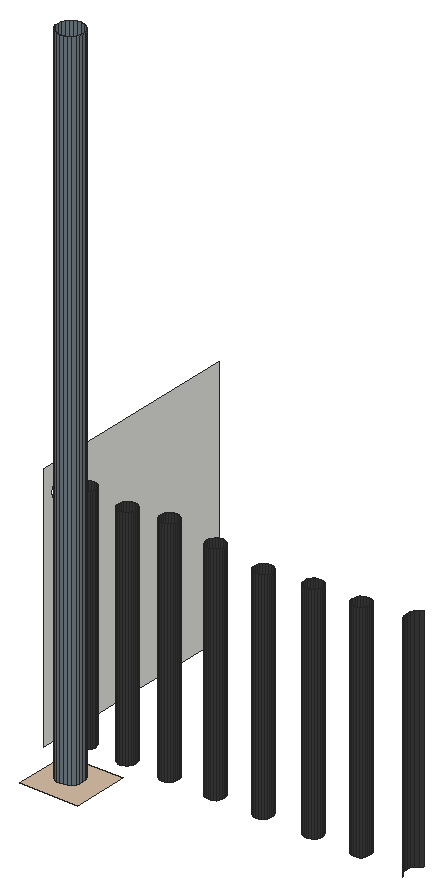
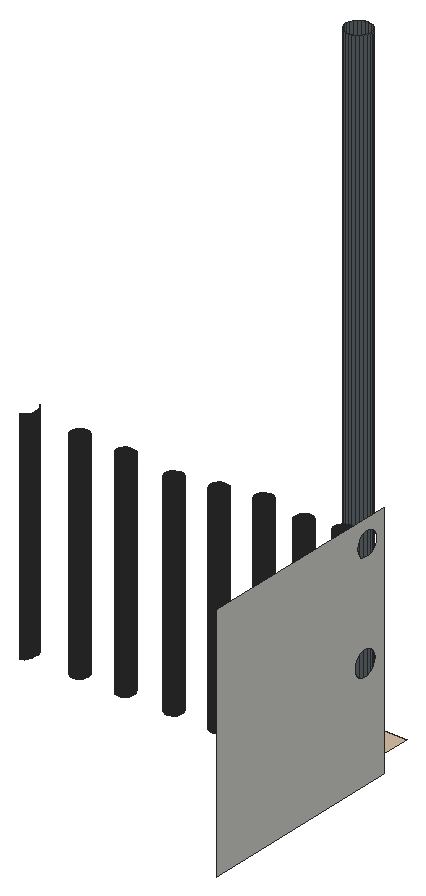
# SketchUp Ruby script. Lengths in inches.
U = 1.inch
M = Sketchup.active_model
def pt(a) = Geom::Point3d.new(a.map { |v| v * U })
def face(e, loops, mat)
  f = e.add_face(loops[0].map { |a| pt(a) })
  loops[1..].each { |l| e.add_face(l.map { |a| pt(a) }).erase! }
  f.material = f.back_material = mat if mat
  f
end
# faces: each face lists its corners as indices into pts; further lists are holes
def faces(e, pts, list, mat = nil) = list.each { |f| face(e, (f[0].is_a?(Array) ? f : [f]).map { |l| l.map { |i| pts[i] } }, mat) }
# xy, xz, yz: faces in a plane at the given z, y or x. An outline is a flat list of corners, or four numbers for a rectangle; further outlines are holes
def ring(l) = l.size == 4 ? [[l[0], l[1]], [l[2], l[1]], [l[2], l[3]], [l[0], l[3]]] : l.each_slice(2).to_a
def flat(e, list, mat, &to3) = list.each { |f| face(e, (f[0].is_a?(Array) ? f : [f]).map { |l| ring(l).map { |u, v| to3.(u, v) } }, mat) }
def xy(e, z, list, mat = nil) = flat(e, list, mat) { |x, y| [x, y, z] }
def xz(e, y, list, mat = nil) = flat(e, list, mat) { |x, z| [x, y, z] }
def yz(e, x, list, mat = nil) = flat(e, list, mat) { |y, z| [x, y, z] }
def lines(e, pts, list) = list.each { |a, b| e.add_line(pt(pts[a]), pt(pts[b])) }
# prism: a flat outline (further loops are holes) pulled along v
def prism(e, loops, v, mat = nil)
  f = face(e, loops, mat); d = Geom::Vector3d.new(v.map { |x| x * U })
  f.pushpull(f.normal.samedirection?(d) ? d.length : -d.length)
end
def box(e, o, s, mat = nil) = prism(e, [[o, [o[0] + s[0], o[1], o[2]], [o[0] + s[0], o[1] + s[1], o[2]], [o[0], o[1] + s[1], o[2]]]], [0, 0, s[2]], mat)
def at(x, y, z, deg = 0) = Geom::Transformation.translation(pt([x, y, z])) * Geom::Transformation.rotation(ORIGIN, Z_AXIS, deg.degrees)
def axes(o, x, y, z) = Geom::Transformation.new([*x, 0, *y, 0, *z, 0, *pt(o).to_a, 1])
def part(name) = M.definitions.add(name)
# library, detail: a bought-in or finely detailed component or shape, given as its bounding box
def library(name, o, s) = part(name).tap { |d| box(d.entities, o, s) }
def detail(e, o, s) = box(e.add_group.entities, o, s)
def put(e, d, t, mat = nil) = e.add_instance(d, t).tap { |i| i.material = mat if mat }
def group(e, t, mat = nil) = e.add_group.tap { |g| g.transformation = t; g.material = mat if mat }.entities
root = M.entities
M.materials.add("[Color M07]").color = [58, 58, 58]
M.materials.add("[Formica Laminate Light]").color = [213, 189, 164]
M.materials.add("[Formica Speckled Grey]").color = [112, 125, 132]
xy(root,479.18,[[50.05,85.59,49.68,85.64,49.33,85.79,49.03,86.02,48.81,86.3125,48.66,86.66,48.61,87.03,48.66,87.4,48.81,87.75,49.03,88.05,49.33,88.28,49.68,88.42,50.05,88.47,50.42,88.42,50.77,88.28,51.07,88.05,51.3,87.75,51.4375,87.4,51.49,87.03,51.4375,86.66,51.3,86.3125,51.07,86.02,50.77,85.79,50.42,85.64],[47.49,91.47,47.23,91.5,46.99,91.6,46.78,91.76,46.62,91.97,46.52,92.21,46.49,92.47,46.52,92.73,46.62,92.97,46.78,93.18,46.99,93.33,47.23,93.43,47.49,93.47,47.74,93.43,47.99,93.33,48.19,93.18,48.35,92.97,48.45,92.73,48.49,92.47,48.45,92.21,48.35,91.97,48.19,91.76,47.99,91.6,47.74,91.5],[52.05,91.47,51.79,91.5,51.55,91.6,51.34,91.76,51.18,91.97,51.08,92.21,51.05,92.47,51.08,92.73,51.18,92.97,51.34,93.18,51.55,93.33,51.79,93.43,52.05,93.47,52.31,93.43,52.55,93.33,52.76,93.18,52.91,92.97,53.01,92.73,53.05,92.47,53.01,92.21,52.91,91.97,52.76,91.76,52.55,91.6,52.31,91.5],[56.74,91.47,56.48,91.5,56.24,91.6,56.03,91.76,55.87,91.97,55.77,92.21,55.74,92.47,55.77,92.73,55.87,92.97,56.03,93.18,56.24,93.33,56.48,93.43,56.74,93.47,56.99,93.43,57.24,93.33,57.44,93.18,57.6,92.97,57.7,92.73,57.74,92.47,57.7,92.21,57.6,91.97,57.44,91.76,57.24,91.6,56.99,91.5],[61.92,91.47,61.66,91.5,61.42,91.6,61.22,91.76,61.06,91.97,60.96,92.21,60.92,92.47,60.96,92.73,61.06,92.97,61.22,93.18,61.42,93.33,61.66,93.43,61.92,93.47,62.18,93.43,62.42,93.33,62.63,93.18,62.79,92.97,62.89,92.73,62.92,92.47,62.89,92.21,62.79,91.97,62.63,91.76,62.42,91.6,62.18,91.5],
  [67.24,91.47,66.98,91.5,66.74,91.6,66.53,91.76,66.37,91.97,66.27,92.21,66.24,92.47,66.27,92.73,66.37,92.97,66.53,93.18,66.74,93.33,66.98,93.43,67.24,93.47,67.49,93.43,67.74,93.33,67.94,93.18,68.1,92.97,68.2,92.73,68.24,92.47,68.2,92.21,68.1,91.97,67.94,91.76,67.74,91.6,67.49,91.5],[72.86,91.47,72.6,91.5,72.36,91.6,72.15,91.76,71.99,91.97,71.89,92.21,71.86,92.47,71.89,92.73,71.99,92.97,72.15,93.18,72.36,93.33,72.6,93.43,72.86,93.47,73.12,93.43,73.36,93.33,73.57,93.18,73.73,92.97,73.83,92.73,73.86,92.47,73.83,92.21,73.73,91.97,73.57,91.76,73.36,91.6,73.12,91.5],[78.17,91.47,77.91,91.5,77.67,91.6,77.47,91.76,77.31,91.97,77.21,92.21,77.17,92.47,77.21,92.73,77.31,92.97,77.47,93.18,77.67,93.33,77.91,93.43,78.17,93.47,78.43,93.43,78.67,93.33,78.88,93.18,79.04,92.97,79.14,92.73,79.17,92.47,79.14,92.21,79.04,91.97,78.88,91.76,78.67,91.6,78.43,91.5]])
xy(root,479.18,[[[47.29,83.48,53.75,89.73],[50.05,85.59,49.68,85.64,49.33,85.79,49.03,86.02,48.81,86.3125,48.66,86.66,48.61,87.03,48.66,87.4,48.81,87.75,49.03,88.05,49.33,88.28,49.68,88.42,50.05,88.47,50.42,88.42,50.77,88.28,51.07,88.05,51.3,87.75,51.4375,87.4,51.49,87.03,51.4375,86.66,51.3,86.3125,51.07,86.02,50.77,85.79,50.42,85.64]]],"[Formica Laminate Light]")
yz(root,44.94,[[[89.73,479.18,114.1,506.99],[92.45,490.42,92.06,490.47,91.7,490.62,91.39,490.86,91.15,491.17,91,491.53,90.95,491.92,91,492.31,91.15,492.67,91.39,492.98,91.7,493.22,92.06,493.37,92.45,493.42,92.84,493.37,93.2,493.22,93.51,492.98,93.75,492.67,93.9,492.31,93.95,491.92,93.9,491.53,93.75,491.17,93.51,490.86,93.2,490.62,92.84,490.47],[92.15,502.86,91.77,502.91,91.43,503.05,91.13,503.28,90.9,503.58,90.76,503.92,90.71,504.3,90.76,504.67,90.9,505.01,91.13,505.3125,91.43,505.54,91.77,505.68,92.15,505.73,92.52,505.68,92.87,505.54,93.16,505.3125,93.39,505.01,93.53,504.67,93.58,504.3,93.53,503.92,93.39,503.58,93.16,503.28,92.87,503.05,92.52,502.91]]])
p = [[49.33,85.79,479.18],[49.68,85.64,479.18],[49.68,85.64,554.07],[49.33,85.79,554.07],[50.05,85.59,479.18],[50.05,85.59,554.07],
  [50.42,85.64,479.18],[50.42,85.64,554.07],[50.77,85.79,479.18],[50.77,85.79,554.07],[50.46,85.66,554.07],[49.03,86.02,479.18],
  [49.03,86.02,554.07],[51.07,86.02,479.18],[51.07,86.02,554.07],[48.81,86.3125,479.18],[48.81,86.3125,554.07],[51.3,86.3125,479.18],
  [51.3,86.3125,554.07],[48.66,86.66,479.18],[48.66,86.66,554.07],[51.4375,86.66,479.18],[51.4375,86.66,554.07],[48.61,87.03,479.18],
  [48.61,87.03,554.07],[51.49,87.03,479.18],[51.49,87.03,554.07],[48.66,87.4,479.18],[48.66,87.4,554.07],[51.4375,87.4,479.18],
  [51.4375,87.4,554.07],[48.81,87.75,479.18],[48.81,87.75,554.07],[51.3,87.75,479.18],[51.3,87.75,554.07],[49.03,88.05,479.18],
  [49.03,88.05,554.07],[51.07,88.05,479.18],[51.07,88.05,554.07],[49.33,88.28,479.18],[49.33,88.28,554.07],[50.77,88.28,479.18],
  [50.77,88.28,554.07],[49.68,88.42,479.18],[49.68,88.42,554.07],[50.42,88.42,479.18],[50.42,88.42,554.07],[50.46,88.4,554.07],
  [50.05,88.47,479.18],[50.05,88.47,554.07],[83.49,91.66,479.18],[83.74,91.33,479.18],[83.74,91.33,504.8],[83.49,91.66,504.8],
  [46.99,91.6,479.18],[47.23,91.5,479.18],[47.23,91.5,505.01],[46.99,91.6,505.01],[47.49,91.47,479.18],[47.49,91.47,505.01],
  [47.74,91.5,479.18],[47.74,91.5,505.01],[47.99,91.6,479.18],[47.99,91.6,505.01],[51.55,91.6,479.18],[51.79,91.5,479.18],
  [51.79,91.5,504.49],[51.55,91.6,504.49],[52.05,91.47,479.18],[52.05,91.47,504.49],[52.31,91.5,479.18],[52.31,91.5,504.49],
  [52.55,91.6,479.18],[52.55,91.6,504.49],[56.24,91.6,479.18],[56.48,91.5,479.18],[56.48,91.5,505.01],[56.24,91.6,505.01],
  [56.74,91.47,479.18],[56.74,91.47,505.01],[56.99,91.5,479.18],[56.99,91.5,505.01],[57.24,91.6,479.18],[57.24,91.6,505.01],
  [61.42,91.6,479.18],[61.66,91.5,479.18],[61.66,91.5,504.3],[61.42,91.6,504.3],[61.92,91.47,479.18],[61.92,91.47,504.3],
  [62.18,91.5,479.18],[62.18,91.5,504.3],[62.42,91.6,479.18],[62.42,91.6,504.3],[66.74,91.6,479.18],[66.98,91.5,479.18],
  [66.98,91.5,503.62],[66.74,91.6,503.62],[67.24,91.47,479.18],[67.24,91.47,503.62],[67.49,91.5,479.18],[67.49,91.5,503.62],
  [67.74,91.6,479.18],[67.74,91.6,503.62],[72.36,91.6,479.18],[72.6,91.5,479.18],[72.6,91.5,504.12],[72.36,91.6,504.12],
  [72.86,91.47,479.18],[72.86,91.47,504.12],[73.12,91.5,479.18],[73.12,91.5,504.12],[73.36,91.6,479.18],[73.36,91.6,504.12],
  [77.67,91.6,479.18],[77.91,91.5,479.18],[77.91,91.5,504.18],[77.67,91.6,504.18],[78.17,91.47,479.18],[78.17,91.47,504.18],
  [78.43,91.5,479.18],[78.43,91.5,504.18],[78.67,91.6,479.18],[78.67,91.6,504.18],[46.78,91.76,479.18],[46.78,91.76,505.01],
  [48.19,91.76,479.18],[48.19,91.76,505.01],[51.34,91.76,479.18],[51.34,91.76,504.49],[52.76,91.76,479.18],[52.76,91.76,504.49],
  [56.03,91.76,479.18],[56.03,91.76,505.01],[57.44,91.76,479.18],[57.44,91.76,505.01],[61.22,91.76,479.18],[61.22,91.76,504.3],
  [62.63,91.76,479.18],[62.63,91.76,504.3],[66.53,91.76,479.18],[66.53,91.76,503.62],[67.94,91.76,479.18],[67.94,91.76,503.62],
  [72.15,91.76,479.18],[72.15,91.76,504.12],[73.57,91.76,479.18],[73.57,91.76,504.12],[77.47,91.76,479.18],[77.47,91.76,504.18],
  [78.88,91.76,479.18],[78.88,91.76,504.18],[83.34,92.03,479.18],[83.34,92.03,504.8],[46.62,91.97,479.18],[46.62,91.97,505.01],
  [48.35,91.97,479.18],[48.35,91.97,505.01],[51.18,91.97,479.18],[51.18,91.97,504.49],[52.91,91.97,479.18],[52.91,91.97,504.49],
  [55.87,91.97,479.18],[55.87,91.97,505.01],[57.6,91.97,479.18],[57.6,91.97,505.01],[61.06,91.97,479.18],[61.06,91.97,504.3],
  [62.79,91.97,479.18],[62.79,91.97,504.3],[66.37,91.97,479.18],[66.37,91.97,503.62],[68.1,91.97,479.18],[68.1,91.97,503.62],
  [71.99,91.97,479.18],[71.99,91.97,504.12],[73.73,91.97,479.18],[73.73,91.97,504.12],[77.31,91.97,479.18],[77.31,91.97,504.18],
  [79.04,91.97,479.18],[79.04,91.97,504.18],[46.52,92.21,479.18],[46.52,92.21,505.01],[48.45,92.21,479.18],[48.45,92.21,505.01],
  [51.08,92.21,479.18],[51.08,92.21,504.49],[53.01,92.21,479.18],[53.01,92.21,504.49],[55.77,92.21,479.18],[55.77,92.21,505.01],
  [57.7,92.21,479.18],[57.7,92.21,505.01],[60.96,92.21,479.18],[60.96,92.21,504.3],[62.89,92.21,479.18],[62.89,92.21,504.3],
  [66.27,92.21,479.18],[66.27,92.21,503.62],[68.2,92.21,479.18],[68.2,92.21,503.62],[71.89,92.21,479.18],[71.89,92.21,504.12],
  [73.83,92.21,479.18],[73.83,92.21,504.12],[77.21,92.21,479.18],[77.21,92.21,504.18],[79.14,92.21,479.18],[79.14,92.21,504.18],
  [83.28,92.4375,479.18],[83.28,92.4375,504.8],[46.49,92.47,479.18],[46.49,92.47,505.01],[48.49,92.47,479.18],[48.49,92.47,505.01],
  [51.05,92.47,479.18],[51.05,92.47,504.49],[53.05,92.47,479.18],[53.05,92.47,504.49],[55.74,92.47,479.18],[55.74,92.47,505.01],
  [57.74,92.47,479.18],[57.74,92.47,505.01],[60.92,92.47,479.18],[60.92,92.47,504.3],[62.92,92.47,479.18],[62.92,92.47,504.3],
  [66.24,92.47,479.18],[66.24,92.47,503.62],[68.24,92.47,479.18],[68.24,92.47,503.62],[71.86,92.47,479.18],[71.86,92.47,504.12],
  [73.86,92.47,479.18],[73.86,92.47,504.12],[77.17,92.47,479.18],[77.17,92.47,504.18],[79.17,92.47,479.18],[79.17,92.47,504.18],
  [83.34,92.84,479.18],[83.34,92.84,504.8],[46.52,92.73,479.18],[46.52,92.73,505.01],[48.45,92.73,479.18],[48.45,92.73,505.01],
  [51.08,92.73,479.18],[51.08,92.73,504.49],[53.01,92.73,479.18],[53.01,92.73,504.49],[55.77,92.73,479.18],[55.77,92.73,505.01],
  [57.7,92.73,479.18],[57.7,92.73,505.01],[60.96,92.73,479.18],[60.96,92.73,504.3],[62.89,92.73,479.18],[62.89,92.73,504.3],
  [66.27,92.73,479.18],[66.27,92.73,503.62],[68.2,92.73,479.18],[68.2,92.73,503.62],[71.89,92.73,479.18],[71.89,92.73,504.12],
  [73.83,92.73,479.18],[73.83,92.73,504.12],[77.21,92.73,479.18],[77.21,92.73,504.18],[79.14,92.73,479.18],[79.14,92.73,504.18],
  [46.62,92.97,479.18],[46.62,92.97,505.01],[48.35,92.97,479.18],[48.35,92.97,505.01],[51.18,92.97,479.18],[51.18,92.97,504.49],
  [52.91,92.97,479.18],[52.91,92.97,504.49],[55.87,92.97,479.18],[55.87,92.97,505.01],[57.6,92.97,479.18],[57.6,92.97,505.01],
  [61.06,92.97,479.18],[61.06,92.97,504.3],[62.79,92.97,479.18],[62.79,92.97,504.3],[66.37,92.97,479.18],[66.37,92.97,503.62],
  [68.1,92.97,479.18],[68.1,92.97,503.62],[71.99,92.97,479.18],[71.99,92.97,504.12],[73.73,92.97,479.18],[73.73,92.97,504.12],
  [77.31,92.97,479.18],[77.31,92.97,504.18],[79.04,92.97,479.18],[79.04,92.97,504.18],[83.49,93.22,479.18],[83.49,93.22,504.8],
  [46.78,93.18,479.18],[46.78,93.18,505.01],[48.19,93.18,479.18],[48.19,93.18,505.01],[51.34,93.18,479.18],[51.34,93.18,504.49],
  [52.76,93.18,479.18],[52.76,93.18,504.49],[56.03,93.18,479.18],[56.03,93.18,505.01],[57.44,93.18,479.18],[57.44,93.18,505.01],
  [61.22,93.18,479.18],[61.22,93.18,504.3],[62.63,93.18,479.18],[62.63,93.18,504.3],[66.53,93.18,479.18],[66.53,93.18,503.62],
  [67.94,93.18,479.18],[67.94,93.18,503.62],[72.15,93.18,479.18],[72.15,93.18,504.12],[73.57,93.18,479.18],[73.57,93.18,504.12],
  [77.47,93.18,479.18],[77.47,93.18,504.18],[78.88,93.18,479.18],[78.88,93.18,504.18],[46.99,93.33,479.18],[46.99,93.33,505.01],
  [47.99,93.33,479.18],[47.99,93.33,505.01],[51.55,93.33,479.18],[51.55,93.33,504.49],[52.55,93.33,479.18],[52.55,93.33,504.49],
  [56.24,93.33,479.18],[56.24,93.33,505.01],[57.24,93.33,479.18],[57.24,93.33,505.01],[61.42,93.33,479.18],[61.42,93.33,504.3],
  [62.42,93.33,479.18],[62.42,93.33,504.3],[66.74,93.33,479.18],[66.74,93.33,503.62],[67.74,93.33,479.18],[67.74,93.33,503.62],
  [72.36,93.33,479.18],[72.36,93.33,504.12],[73.36,93.33,479.18],[73.36,93.33,504.12],[77.67,93.33,479.18],[77.67,93.33,504.18],
  [78.67,93.33,479.18],[78.67,93.33,504.18],[83.74,93.54,479.18],[83.74,93.54,504.8],[47.23,93.43,479.18],[47.12,93.39,505.01],
  [47.23,93.43,505.01],[47.74,93.43,479.18],[47.74,93.43,505.01],[47.85,93.39,505.01],[51.79,93.43,479.18],[51.79,93.43,504.49],
  [52.31,93.43,479.18],[52.31,93.43,504.49],[56.48,93.43,479.18],[56.37,93.39,505.01],[56.48,93.43,505.01],[56.99,93.43,479.18],
  [56.99,93.43,505.01],[57.1,93.39,505.01],[61.66,93.43,479.18],[61.66,93.43,504.3],[62.18,93.43,479.18],[62.18,93.43,504.3],
  [66.98,93.43,479.18],[66.98,93.43,503.62],[67.49,93.43,479.18],[67.49,93.43,503.62],[72.6,93.43,479.18],[72.6,93.43,504.12],
  [73.12,93.43,479.18],[73.12,93.43,504.12],[77.91,93.43,479.18],[77.91,93.43,504.18],[78.43,93.43,479.18],[78.43,93.43,504.18],
  [47.49,93.47,479.18],[47.49,93.47,505.01],[52.05,93.47,479.18],[52.05,93.47,504.49],[56.74,93.47,479.18],[56.74,93.47,505.01],
  [61.92,93.47,479.18],[61.92,93.47,504.3],[67.24,93.47,479.18],[67.24,93.47,503.62],[72.86,93.47,479.18],[72.86,93.47,504.12],
  [78.17,93.47,479.18],[78.17,93.47,504.18],[84.0625,93.79,479.18],[84.0625,93.79,504.8]]
faces(root,p,[[0,1,2,3],[1,4,5,2],[4,6,7,5],[6,8,9,10,7],[11,0,3,12],[8,13,14,9],[15,11,12,16],[13,17,18,14],
  [19,15,16,20],[17,21,22,18],[23,19,20,24],[21,25,26,22],[27,23,24,28],[25,29,30,26],[31,27,28,32],[29,33,34,30],
  [35,31,32,36],[33,37,38,34],[39,35,36,40],[37,41,42,38],[43,39,40,44],[41,45,46,47,42],[48,43,44,49],[45,48,49,46]],"[Formica Speckled Grey]")
faces(root,p,[[50,51,52,53],[54,55,56,57],[55,58,59,56],[58,60,61,59],[60,62,63,61],[64,65,66,67],[65,68,69,66],[68,70,71,69],
  [70,72,73,71],[74,75,76,77],[75,78,79,76],[78,80,81,79],[80,82,83,81],[84,85,86,87],[85,88,89,86],[88,90,91,89],
  [90,92,93,91],[94,95,96,97],[95,98,99,96],[98,100,101,99],[100,102,103,101],[104,105,106,107],[105,108,109,106],[108,110,111,109],
  [110,112,113,111],[114,115,116,117],[115,118,119,116],[118,120,121,119],[120,122,123,121],[124,54,57,125],[62,126,127,63],[128,64,67,129],
  [72,130,131,73],[132,74,77,133],[82,134,135,83],[136,84,87,137],[92,138,139,93],[140,94,97,141],[102,142,143,103],[144,104,107,145],
  [112,146,147,113],[148,114,117,149],[122,150,151,123],[152,50,53,153],[154,124,125,155],[126,156,157,127],[158,128,129,159],[130,160,161,131],
  [162,132,133,163],[134,164,165,135],[166,136,137,167],[138,168,169,139],[170,140,141,171],[142,172,173,143],[174,144,145,175],[146,176,177,147],
  [178,148,149,179],[150,180,181,151],[182,154,155,183],[156,184,185,157],[186,158,159,187],[160,188,189,161],[190,162,163,191],[164,192,193,165],
  [194,166,167,195],[168,196,197,169],[198,170,171,199],[172,200,201,173],[202,174,175,203],[176,204,205,177],[206,178,179,207],[180,208,209,181],
  [210,152,153,211],[212,182,183,213],[184,214,215,185],[216,186,187,217],[188,218,219,189],[220,190,191,221],[192,222,223,193],[224,194,195,225],
  [196,226,227,197],[228,198,199,229],[200,230,231,201],[232,202,203,233],[204,234,235,205],[236,206,207,237],[208,238,239,209],[240,210,211,241],
  [242,212,213,243],[214,244,245,215],[246,216,217,247],[218,248,249,219],[250,220,221,251],[222,252,253,223],[254,224,225,255],[226,256,257,227],
  [258,228,229,259],[230,260,261,231],[262,232,233,263],[234,264,265,235],[266,236,237,267],[238,268,269,239],[270,242,243,271],[244,272,273,245],
  [274,246,247,275],[248,276,277,249],[278,250,251,279],[252,280,281,253],[282,254,255,283],[256,284,285,257],[286,258,259,287],[260,288,289,261],
  [290,262,263,291],[264,292,293,265],[294,266,267,295],[268,296,297,269],[298,240,241,299],[300,270,271,301],[272,302,303,273],[304,274,275,305],
  [276,306,307,277],[308,278,279,309],[280,310,311,281],[312,282,283,313],[284,314,315,285],[316,286,287,317],[288,318,319,289],[320,290,291,321],
  [292,322,323,293],[324,294,295,325],[296,326,327,297],[328,300,301,329],[302,330,331,303],[332,304,305,333],[306,334,335,307],[336,308,309,337],
  [310,338,339,311],[340,312,313,341],[314,342,343,315],[344,316,317,345],[318,346,347,319],[348,320,321,349],[322,350,351,323],[352,324,325,353],
  [326,354,355,327],[356,298,299,357],[358,328,329,359,360],[330,361,362,363,331],[364,332,333,365],[334,366,367,335],[368,336,337,369,370],[338,371,372,373,339],
  [374,340,341,375],[342,376,377,343],[378,344,345,379],[346,380,381,347],[382,348,349,383],[350,384,385,351],[386,352,353,387],[354,388,389,355],
  [390,358,360,391],[361,390,391,362],[392,364,365,393],[366,392,393,367],[394,368,370,395],[371,394,395,372],[396,374,375,397],[376,396,397,377],
  [398,378,379,399],[380,398,399,381],[400,382,383,401],[384,400,401,385],[402,386,387,403],[388,402,403,389],[404,356,357,405]],"[Color M07]")
